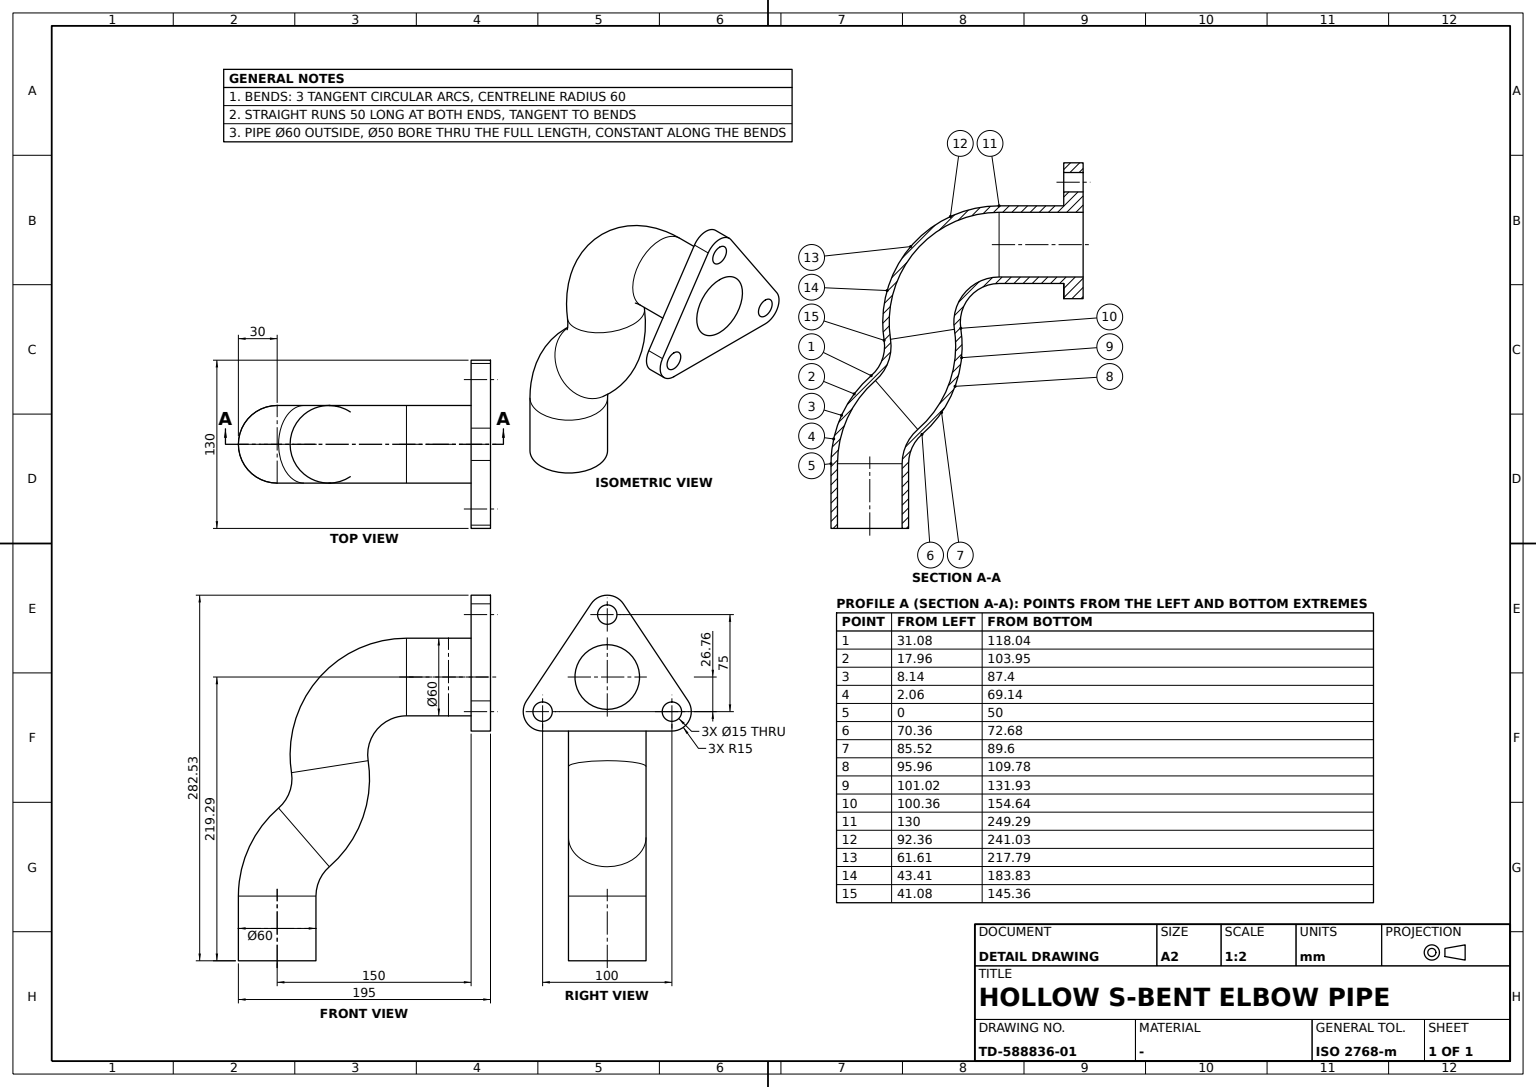
ISO-10303-21;
HEADER;
FILE_DESCRIPTION((''),'2;1');
FILE_NAME('','',(''),(''),'','','');
FILE_SCHEMA(('AUTOMOTIVE_DESIGN'));
ENDSEC;
DATA;
#1=APPLICATION_CONTEXT('');
#2=PRODUCT_CONTEXT('',#1,'mechanical');
#3=PRODUCT('','','',(#2));
#4=PRODUCT_DEFINITION_FORMATION('','',#3);
#5=PRODUCT_DEFINITION_CONTEXT('',#1,'design');
#6=PRODUCT_DEFINITION('','',#4,#5);
#7=PRODUCT_DEFINITION_SHAPE('','',#6);
#8=(LENGTH_UNIT()NAMED_UNIT(*)SI_UNIT(.MILLI.,.METRE.));
#9=(NAMED_UNIT(*)PLANE_ANGLE_UNIT()SI_UNIT($,.RADIAN.));
#10=(NAMED_UNIT(*)SI_UNIT($,.STERADIAN.)SOLID_ANGLE_UNIT());
#11=UNCERTAINTY_MEASURE_WITH_UNIT(LENGTH_MEASURE(0.005),#8,'distance_accuracy_value','');
#12=(GEOMETRIC_REPRESENTATION_CONTEXT(3)GLOBAL_UNCERTAINTY_ASSIGNED_CONTEXT((#11))GLOBAL_UNIT_ASSIGNED_CONTEXT((#8,#9,#10))REPRESENTATION_CONTEXT('',''));
#13=CARTESIAN_POINT('',(-50.,165.,200.025861));
#14=VERTEX_POINT('',#13);
#15=CARTESIAN_POINT('',(-50.,165.,192.525861));
#16=DIRECTION('',(0.,1.,0.));
#17=DIRECTION('',(0.,0.,1.));
#18=AXIS2_PLACEMENT_3D('',#15,#16,#17);
#19=CIRCLE('',#18,7.5);
#20=EDGE_CURVE('',#14,#14,#19,.T.);
#21=ORIENTED_EDGE('',*,*,#20,.T.);
#22=EDGE_LOOP('',(#21));
#23=FACE_BOUND('',#22,.T.);
#24=CARTESIAN_POINT('',(-50.,150.,200.025861));
#25=VERTEX_POINT('',#24);
#26=CARTESIAN_POINT('',(-50.,150.,192.525861));
#27=AXIS2_PLACEMENT_3D('',#26,#16,#17);
#28=CIRCLE('',#27,7.5);
#29=EDGE_CURVE('',#25,#25,#28,.T.);
#30=ORIENTED_EDGE('',*,*,#29,.F.);
#31=EDGE_LOOP('',(#30));
#32=FACE_BOUND('',#31,.T.);
#33=CARTESIAN_POINT('',(-50.,157.5,192.525861));
#34=DIRECTION('',(-1.,0.,0.));
#35=AXIS2_PLACEMENT_3D('',#33,#16,#34);
#36=CYLINDRICAL_SURFACE('',#35,7.5);
#37=ADVANCED_FACE('',(#23,#32),#36,.F.);
#38=CARTESIAN_POINT('',(0.,100.,194.285048));
#39=VERTEX_POINT('',#38);
#40=CARTESIAN_POINT('',(0.,100.,219.285048));
#41=DIRECTION('',(0.,-1.,0.));
#42=DIRECTION('',(0.,0.,-1.));
#43=AXIS2_PLACEMENT_3D('',#40,#41,#42);
#44=CIRCLE('',#43,25.);
#45=EDGE_CURVE('',#39,#39,#44,.T.);
#46=ORIENTED_EDGE('',*,*,#45,.T.);
#47=EDGE_LOOP('',(#46));
#48=FACE_BOUND('',#47,.T.);
#49=CARTESIAN_POINT('',(0.,165.,244.285048));
#50=VERTEX_POINT('',#49);
#51=CARTESIAN_POINT('',(0.,165.,219.285048));
#52=AXIS2_PLACEMENT_3D('',#51,#16,#17);
#53=CIRCLE('',#52,25.);
#54=EDGE_CURVE('',#50,#50,#53,.T.);
#55=ORIENTED_EDGE('',*,*,#54,.T.);
#56=EDGE_LOOP('',(#55));
#57=FACE_BOUND('',#56,.T.);
#58=CARTESIAN_POINT('',(0.,125.,219.285048));
#59=DIRECTION('',(1.,0.,0.));
#60=AXIS2_PLACEMENT_3D('',#58,#41,#59);
#61=CYLINDRICAL_SURFACE('',#60,25.);
#62=ADVANCED_FACE('',(#48,#57),#61,.F.);
#63=CARTESIAN_POINT('',(0.,4.357283,114.256424));
#64=VERTEX_POINT('',#63);
#65=CARTESIAN_POINT('',(0.,20.722788,95.357476));
#66=DIRECTION('',(0.,0.75595793,0.654620202));
#67=DIRECTION('',(0.,-0.654620202,0.75595793));
#68=AXIS2_PLACEMENT_3D('',#65,#66,#67);
#69=CIRCLE('',#68,25.);
#70=EDGE_CURVE('',#64,#64,#69,.F.);
#71=ORIENTED_EDGE('',*,*,#70,.F.);
#72=EDGE_LOOP('',(#71));
#73=FACE_BOUND('',#72,.T.);
#74=CARTESIAN_POINT('',(-25.,0.,50.));
#75=VERTEX_POINT('',#74);
#76=CARTESIAN_POINT('',(0.,0.,50.));
#77=AXIS2_PLACEMENT_3D('',#76,#42,#34);
#78=CIRCLE('',#77,25.);
#79=EDGE_CURVE('',#75,#75,#78,.T.);
#80=ORIENTED_EDGE('',*,*,#79,.T.);
#81=EDGE_LOOP('',(#80));
#82=FACE_BOUND('',#81,.T.);
#83=CARTESIAN_POINT('',(0.,60.,50.));
#84=AXIS2_PLACEMENT_3D('',#83,#59,#67);
#85=TOROIDAL_SURFACE('',#84,60.,25.);
#86=ADVANCED_FACE('',(#73,#82),#85,.F.);
#87=CARTESIAN_POINT('',(50.,165.,200.025861));
#88=VERTEX_POINT('',#87);
#89=CARTESIAN_POINT('',(50.,165.,192.525861));
#90=AXIS2_PLACEMENT_3D('',#89,#16,#17);
#91=CIRCLE('',#90,7.5);
#92=EDGE_CURVE('',#88,#88,#91,.T.);
#93=ORIENTED_EDGE('',*,*,#92,.F.);
#94=EDGE_LOOP('',(#93));
#95=FACE_BOUND('',#94,.T.);
#96=ORIENTED_EDGE('',*,*,#20,.F.);
#97=EDGE_LOOP('',(#96));
#98=FACE_BOUND('',#97,.T.);
#99=CARTESIAN_POINT('',(0.,165.,275.025861));
#100=VERTEX_POINT('',#99);
#101=CARTESIAN_POINT('',(0.,165.,267.525861));
#102=AXIS2_PLACEMENT_3D('',#101,#16,#17);
#103=CIRCLE('',#102,7.5);
#104=EDGE_CURVE('',#100,#100,#103,.T.);
#105=ORIENTED_EDGE('',*,*,#104,.F.);
#106=EDGE_LOOP('',(#105));
#107=FACE_BOUND('',#106,.T.);
#108=ORIENTED_EDGE('',*,*,#54,.F.);
#109=EDGE_LOOP('',(#108));
#110=FACE_BOUND('',#109,.T.);
#111=CARTESIAN_POINT('',(-50.,165.,177.525861));
#112=VERTEX_POINT('',#111);
#113=CARTESIAN_POINT('',(-62.480754,165.,200.846363));
#114=VERTEX_POINT('',#113);
#115=CIRCLE('',#18,15.);
#116=EDGE_CURVE('',#112,#114,#115,.T.);
#117=ORIENTED_EDGE('',*,*,#116,.T.);
#118=CARTESIAN_POINT('',(-12.480754,165.,275.846363));
#119=VERTEX_POINT('',#118);
#120=CARTESIAN_POINT('',(-135.954229,165.,90.636152));
#121=DIRECTION('',(0.554700196,0.,0.832050294));
#122=VECTOR('',#121,1000.);
#123=LINE('',#120,#122);
#124=EDGE_CURVE('',#114,#119,#123,.T.);
#125=ORIENTED_EDGE('',*,*,#124,.T.);
#126=CARTESIAN_POINT('',(12.480754,165.,275.846363));
#127=VERTEX_POINT('',#126);
#128=CIRCLE('',#102,15.);
#129=EDGE_CURVE('',#119,#127,#128,.T.);
#130=ORIENTED_EDGE('',*,*,#129,.T.);
#131=CARTESIAN_POINT('',(62.480754,165.,200.846363));
#132=VERTEX_POINT('',#131);
#133=CARTESIAN_POINT('',(135.954229,165.,90.636152));
#134=DIRECTION('',(0.554700196,0.,-0.832050294));
#135=VECTOR('',#134,1000.);
#136=LINE('',#133,#135);
#137=EDGE_CURVE('',#127,#132,#136,.T.);
#138=ORIENTED_EDGE('',*,*,#137,.T.);
#139=CARTESIAN_POINT('',(50.,165.,177.525861));
#140=VERTEX_POINT('',#139);
#141=CIRCLE('',#90,15.);
#142=EDGE_CURVE('',#132,#140,#141,.T.);
#143=ORIENTED_EDGE('',*,*,#142,.T.);
#144=CARTESIAN_POINT('',(0.,165.,177.525861));
#145=VECTOR('',#34,1000.);
#146=LINE('',#144,#145);
#147=EDGE_CURVE('',#140,#112,#146,.T.);
#148=ORIENTED_EDGE('',*,*,#147,.T.);
#149=EDGE_LOOP('',(#117,#125,#130,#138,#143,#148));
#150=FACE_BOUND('',#149,.T.);
#151=CARTESIAN_POINT('',(0.,165.,0.));
#152=AXIS2_PLACEMENT_3D('',#151,#16,#34);
#153=PLANE('',#152);
#154=ADVANCED_FACE('',(#95,#98,#107,#110,#150),#153,.T.);
#155=CARTESIAN_POINT('',(0.,70.361394,154.642524));
#156=VERTEX_POINT('',#155);
#157=CARTESIAN_POINT('',(0.,40.722788,150.));
#158=DIRECTION('',(0.,0.154750807,-0.987953535));
#159=DIRECTION('',(0.,0.987953535,0.154750807));
#160=AXIS2_PLACEMENT_3D('',#157,#158,#159);
#161=CIRCLE('',#160,30.);
#162=EDGE_CURVE('',#156,#156,#161,.F.);
#163=ORIENTED_EDGE('',*,*,#162,.F.);
#164=EDGE_LOOP('',(#163));
#165=FACE_BOUND('',#164,.T.);
#166=CARTESIAN_POINT('',(0.,1.084182,118.036214));
#167=VERTEX_POINT('',#166);
#168=CIRCLE('',#68,30.);
#169=EDGE_CURVE('',#167,#167,#168,.T.);
#170=ORIENTED_EDGE('',*,*,#169,.T.);
#171=EDGE_LOOP('',(#170));
#172=FACE_BOUND('',#171,.T.);
#173=CARTESIAN_POINT('',(0.,-18.554424,140.714952));
#174=DIRECTION('',(0.,0.654620202,-0.75595793));
#175=AXIS2_PLACEMENT_3D('',#173,#59,#174);
#176=TOROIDAL_SURFACE('',#175,60.,30.);
#177=ADVANCED_FACE('',(#165,#172),#176,.T.);
#178=CARTESIAN_POINT('',(30.,0.,0.));
#179=VERTEX_POINT('',#178);
#180=CARTESIAN_POINT('',(0.,0.,0.));
#181=AXIS2_PLACEMENT_3D('',#180,#17,#59);
#182=CIRCLE('',#181,30.);
#183=EDGE_CURVE('',#179,#179,#182,.T.);
#184=ORIENTED_EDGE('',*,*,#183,.T.);
#185=EDGE_LOOP('',(#184));
#186=FACE_BOUND('',#185,.T.);
#187=CARTESIAN_POINT('',(30.,0.,50.));
#188=VERTEX_POINT('',#187);
#189=AXIS2_PLACEMENT_3D('',#76,#17,#59);
#190=CIRCLE('',#189,30.);
#191=EDGE_CURVE('',#188,#188,#190,.T.);
#192=ORIENTED_EDGE('',*,*,#191,.F.);
#193=EDGE_LOOP('',(#192));
#194=FACE_BOUND('',#193,.T.);
#195=CARTESIAN_POINT('',(0.,0.,25.));
#196=AXIS2_PLACEMENT_3D('',#195,#17,#59);
#197=CYLINDRICAL_SURFACE('',#196,30.);
#198=ADVANCED_FACE('',(#186,#194),#197,.T.);
#199=ORIENTED_EDGE('',*,*,#191,.T.);
#200=EDGE_LOOP('',(#199));
#201=FACE_BOUND('',#200,.T.);
#202=ORIENTED_EDGE('',*,*,#169,.F.);
#203=EDGE_LOOP('',(#202));
#204=FACE_BOUND('',#203,.T.);
#205=TOROIDAL_SURFACE('',#84,60.,30.);
#206=ADVANCED_FACE('',(#201,#204),#205,.T.);
#207=CARTESIAN_POINT('',(0.,65.421626,153.86877));
#208=VERTEX_POINT('',#207);
#209=CIRCLE('',#160,25.);
#210=EDGE_CURVE('',#208,#208,#209,.T.);
#211=ORIENTED_EDGE('',*,*,#210,.T.);
#212=EDGE_LOOP('',(#211));
#213=FACE_BOUND('',#212,.T.);
#214=ORIENTED_EDGE('',*,*,#45,.F.);
#215=EDGE_LOOP('',(#214));
#216=FACE_BOUND('',#215,.T.);
#217=CARTESIAN_POINT('',(0.,100.,159.285048));
#218=AXIS2_PLACEMENT_3D('',#217,#59,#17);
#219=TOROIDAL_SURFACE('',#218,60.,25.);
#220=ADVANCED_FACE('',(#213,#216),#219,.F.);
#221=ORIENTED_EDGE('',*,*,#29,.T.);
#222=EDGE_LOOP('',(#221));
#223=FACE_BOUND('',#222,.T.);
#224=CARTESIAN_POINT('',(50.,150.,177.525861));
#225=VERTEX_POINT('',#224);
#226=CARTESIAN_POINT('',(-50.,150.,177.525861));
#227=VERTEX_POINT('',#226);
#228=CARTESIAN_POINT('',(0.,150.,177.525861));
#229=LINE('',#228,#145);
#230=EDGE_CURVE('',#225,#227,#229,.T.);
#231=ORIENTED_EDGE('',*,*,#230,.F.);
#232=CARTESIAN_POINT('',(62.480754,150.,200.846363));
#233=VERTEX_POINT('',#232);
#234=CARTESIAN_POINT('',(50.,150.,192.525861));
#235=AXIS2_PLACEMENT_3D('',#234,#16,#17);
#236=CIRCLE('',#235,15.);
#237=EDGE_CURVE('',#233,#225,#236,.T.);
#238=ORIENTED_EDGE('',*,*,#237,.F.);
#239=CARTESIAN_POINT('',(12.480754,150.,275.846363));
#240=VERTEX_POINT('',#239);
#241=CARTESIAN_POINT('',(34.745745,150.,242.448878));
#242=LINE('',#241,#135);
#243=EDGE_CURVE('',#240,#233,#242,.T.);
#244=ORIENTED_EDGE('',*,*,#243,.F.);
#245=CARTESIAN_POINT('',(-12.480754,150.,275.846363));
#246=VERTEX_POINT('',#245);
#247=CARTESIAN_POINT('',(0.,150.,267.525861));
#248=AXIS2_PLACEMENT_3D('',#247,#16,#17);
#249=CIRCLE('',#248,15.);
#250=EDGE_CURVE('',#246,#240,#249,.T.);
#251=ORIENTED_EDGE('',*,*,#250,.F.);
#252=CARTESIAN_POINT('',(-62.480754,150.,200.846363));
#253=VERTEX_POINT('',#252);
#254=CARTESIAN_POINT('',(-34.745745,150.,242.448878));
#255=LINE('',#254,#122);
#256=EDGE_CURVE('',#253,#246,#255,.T.);
#257=ORIENTED_EDGE('',*,*,#256,.F.);
#258=CIRCLE('',#27,15.);
#259=EDGE_CURVE('',#227,#253,#258,.T.);
#260=ORIENTED_EDGE('',*,*,#259,.F.);
#261=EDGE_LOOP('',(#231,#238,#244,#251,#257,#260));
#262=FACE_BOUND('',#261,.T.);
#263=CARTESIAN_POINT('',(50.,150.,200.025861));
#264=VERTEX_POINT('',#263);
#265=CIRCLE('',#235,7.5);
#266=EDGE_CURVE('',#264,#264,#265,.T.);
#267=ORIENTED_EDGE('',*,*,#266,.T.);
#268=EDGE_LOOP('',(#267));
#269=FACE_BOUND('',#268,.T.);
#270=CARTESIAN_POINT('',(0.,150.,275.025861));
#271=VERTEX_POINT('',#270);
#272=CIRCLE('',#248,7.5);
#273=EDGE_CURVE('',#271,#271,#272,.T.);
#274=ORIENTED_EDGE('',*,*,#273,.T.);
#275=EDGE_LOOP('',(#274));
#276=FACE_BOUND('',#275,.T.);
#277=CARTESIAN_POINT('',(0.,150.,249.285048));
#278=VERTEX_POINT('',#277);
#279=CARTESIAN_POINT('',(0.,150.,219.285048));
#280=AXIS2_PLACEMENT_3D('',#279,#16,#17);
#281=CIRCLE('',#280,30.);
#282=EDGE_CURVE('',#278,#278,#281,.T.);
#283=ORIENTED_EDGE('',*,*,#282,.T.);
#284=EDGE_LOOP('',(#283));
#285=FACE_BOUND('',#284,.T.);
#286=AXIS2_PLACEMENT_3D('',#279,#16,#59);
#287=PLANE('',#286);
#288=ADVANCED_FACE('',(#223,#262,#269,#276,#285),#287,.F.);
#289=ORIENTED_EDGE('',*,*,#243,.T.);
#290=CARTESIAN_POINT('',(62.480754,157.5,200.846363));
#291=VECTOR('',#16,1000.);
#292=LINE('',#290,#291);
#293=EDGE_CURVE('',#233,#132,#292,.T.);
#294=ORIENTED_EDGE('',*,*,#293,.T.);
#295=ORIENTED_EDGE('',*,*,#137,.F.);
#296=CARTESIAN_POINT('',(12.480754,157.5,275.846363));
#297=LINE('',#296,#291);
#298=EDGE_CURVE('',#240,#127,#297,.T.);
#299=ORIENTED_EDGE('',*,*,#298,.F.);
#300=EDGE_LOOP('',(#289,#294,#295,#299));
#301=FACE_BOUND('',#300,.T.);
#302=DIRECTION('',(0.832050294,0.,0.554700196));
#303=AXIS2_PLACEMENT_3D('',#239,#302,#134);
#304=PLANE('',#303);
#305=ADVANCED_FACE('',(#301),#304,.T.);
#306=ORIENTED_EDGE('',*,*,#259,.T.);
#307=CARTESIAN_POINT('',(-62.480754,157.5,200.846363));
#308=LINE('',#307,#291);
#309=EDGE_CURVE('',#253,#114,#308,.T.);
#310=ORIENTED_EDGE('',*,*,#309,.T.);
#311=ORIENTED_EDGE('',*,*,#116,.F.);
#312=CARTESIAN_POINT('',(-50.,157.5,177.525861));
#313=LINE('',#312,#291);
#314=EDGE_CURVE('',#227,#112,#313,.T.);
#315=ORIENTED_EDGE('',*,*,#314,.F.);
#316=EDGE_LOOP('',(#306,#310,#311,#315));
#317=FACE_BOUND('',#316,.T.);
#318=CYLINDRICAL_SURFACE('',#35,15.);
#319=ADVANCED_FACE('',(#317),#318,.T.);
#320=CARTESIAN_POINT('',(0.,100.,249.285048));
#321=VERTEX_POINT('',#320);
#322=AXIS2_PLACEMENT_3D('',#40,#16,#17);
#323=CIRCLE('',#322,30.);
#324=EDGE_CURVE('',#321,#321,#323,.T.);
#325=ORIENTED_EDGE('',*,*,#324,.F.);
#326=EDGE_LOOP('',(#325));
#327=FACE_BOUND('',#326,.T.);
#328=ORIENTED_EDGE('',*,*,#162,.T.);
#329=EDGE_LOOP('',(#328));
#330=FACE_BOUND('',#329,.T.);
#331=TOROIDAL_SURFACE('',#218,60.,30.);
#332=ADVANCED_FACE('',(#327,#330),#331,.T.);
#333=ORIENTED_EDGE('',*,*,#79,.F.);
#334=EDGE_LOOP('',(#333));
#335=FACE_BOUND('',#334,.T.);
#336=CARTESIAN_POINT('',(25.,0.,0.));
#337=VERTEX_POINT('',#336);
#338=CIRCLE('',#181,25.);
#339=EDGE_CURVE('',#337,#337,#338,.F.);
#340=ORIENTED_EDGE('',*,*,#339,.T.);
#341=EDGE_LOOP('',(#340));
#342=FACE_BOUND('',#341,.T.);
#343=AXIS2_PLACEMENT_3D('',#195,#42,#59);
#344=CYLINDRICAL_SURFACE('',#343,25.);
#345=ADVANCED_FACE('',(#335,#342),#344,.F.);
#346=ORIENTED_EDGE('',*,*,#266,.F.);
#347=EDGE_LOOP('',(#346));
#348=FACE_BOUND('',#347,.T.);
#349=ORIENTED_EDGE('',*,*,#92,.T.);
#350=EDGE_LOOP('',(#349));
#351=FACE_BOUND('',#350,.T.);
#352=CARTESIAN_POINT('',(50.,157.5,192.525861));
#353=AXIS2_PLACEMENT_3D('',#352,#16,#34);
#354=CYLINDRICAL_SURFACE('',#353,7.5);
#355=ADVANCED_FACE('',(#348,#351),#354,.F.);
#356=ORIENTED_EDGE('',*,*,#339,.F.);
#357=EDGE_LOOP('',(#356));
#358=FACE_BOUND('',#357,.T.);
#359=ORIENTED_EDGE('',*,*,#183,.F.);
#360=EDGE_LOOP('',(#359));
#361=FACE_BOUND('',#360,.T.);
#362=PLANE('',#181);
#363=ADVANCED_FACE('',(#358,#361),#362,.F.);
#364=ORIENTED_EDGE('',*,*,#324,.T.);
#365=EDGE_LOOP('',(#364));
#366=FACE_BOUND('',#365,.T.);
#367=ORIENTED_EDGE('',*,*,#282,.F.);
#368=EDGE_LOOP('',(#367));
#369=FACE_BOUND('',#368,.T.);
#370=AXIS2_PLACEMENT_3D('',#58,#16,#59);
#371=CYLINDRICAL_SURFACE('',#370,30.);
#372=ADVANCED_FACE('',(#366,#369),#371,.T.);
#373=ORIENTED_EDGE('',*,*,#70,.T.);
#374=EDGE_LOOP('',(#373));
#375=FACE_BOUND('',#374,.T.);
#376=ORIENTED_EDGE('',*,*,#210,.F.);
#377=EDGE_LOOP('',(#376));
#378=FACE_BOUND('',#377,.T.);
#379=TOROIDAL_SURFACE('',#175,60.,25.);
#380=ADVANCED_FACE('',(#375,#378),#379,.F.);
#381=ORIENTED_EDGE('',*,*,#298,.T.);
#382=ORIENTED_EDGE('',*,*,#129,.F.);
#383=CARTESIAN_POINT('',(-12.480754,157.5,275.846363));
#384=LINE('',#383,#291);
#385=EDGE_CURVE('',#246,#119,#384,.T.);
#386=ORIENTED_EDGE('',*,*,#385,.F.);
#387=ORIENTED_EDGE('',*,*,#250,.T.);
#388=EDGE_LOOP('',(#381,#382,#386,#387));
#389=FACE_BOUND('',#388,.T.);
#390=CARTESIAN_POINT('',(0.,157.5,267.525861));
#391=AXIS2_PLACEMENT_3D('',#390,#16,#34);
#392=CYLINDRICAL_SURFACE('',#391,15.);
#393=ADVANCED_FACE('',(#389),#392,.T.);
#394=CARTESIAN_POINT('',(50.,157.5,177.525861));
#395=LINE('',#394,#291);
#396=EDGE_CURVE('',#225,#140,#395,.T.);
#397=ORIENTED_EDGE('',*,*,#396,.F.);
#398=ORIENTED_EDGE('',*,*,#230,.T.);
#399=ORIENTED_EDGE('',*,*,#314,.T.);
#400=ORIENTED_EDGE('',*,*,#147,.F.);
#401=EDGE_LOOP('',(#397,#398,#399,#400));
#402=FACE_BOUND('',#401,.T.);
#403=AXIS2_PLACEMENT_3D('',#224,#42,#34);
#404=PLANE('',#403);
#405=ADVANCED_FACE('',(#402),#404,.T.);
#406=ORIENTED_EDGE('',*,*,#273,.F.);
#407=EDGE_LOOP('',(#406));
#408=FACE_BOUND('',#407,.T.);
#409=ORIENTED_EDGE('',*,*,#104,.T.);
#410=EDGE_LOOP('',(#409));
#411=FACE_BOUND('',#410,.T.);
#412=CYLINDRICAL_SURFACE('',#391,7.5);
#413=ADVANCED_FACE('',(#408,#411),#412,.F.);
#414=ORIENTED_EDGE('',*,*,#237,.T.);
#415=ORIENTED_EDGE('',*,*,#396,.T.);
#416=ORIENTED_EDGE('',*,*,#142,.F.);
#417=ORIENTED_EDGE('',*,*,#293,.F.);
#418=EDGE_LOOP('',(#414,#415,#416,#417));
#419=FACE_BOUND('',#418,.T.);
#420=CYLINDRICAL_SURFACE('',#353,15.);
#421=ADVANCED_FACE('',(#419),#420,.T.);
#422=ORIENTED_EDGE('',*,*,#309,.F.);
#423=ORIENTED_EDGE('',*,*,#256,.T.);
#424=ORIENTED_EDGE('',*,*,#385,.T.);
#425=ORIENTED_EDGE('',*,*,#124,.F.);
#426=EDGE_LOOP('',(#422,#423,#424,#425));
#427=FACE_BOUND('',#426,.T.);
#428=DIRECTION('',(-0.832050294,0.,0.554700196));
#429=AXIS2_PLACEMENT_3D('',#252,#428,#121);
#430=PLANE('',#429);
#431=ADVANCED_FACE('',(#427),#430,.T.);
#432=CLOSED_SHELL('',(#37,#62,#86,#154,#177,#198,#206,#220,#288,#305,#319,#332,#345,#355,#363,#372,#380,#393,#405,#413,#421,#431));
#433=MANIFOLD_SOLID_BREP('',#432);
#434=ADVANCED_BREP_SHAPE_REPRESENTATION('',(#433),#12);
#435=SHAPE_DEFINITION_REPRESENTATION(#7,#434);
ENDSEC;
END-ISO-10303-21;
